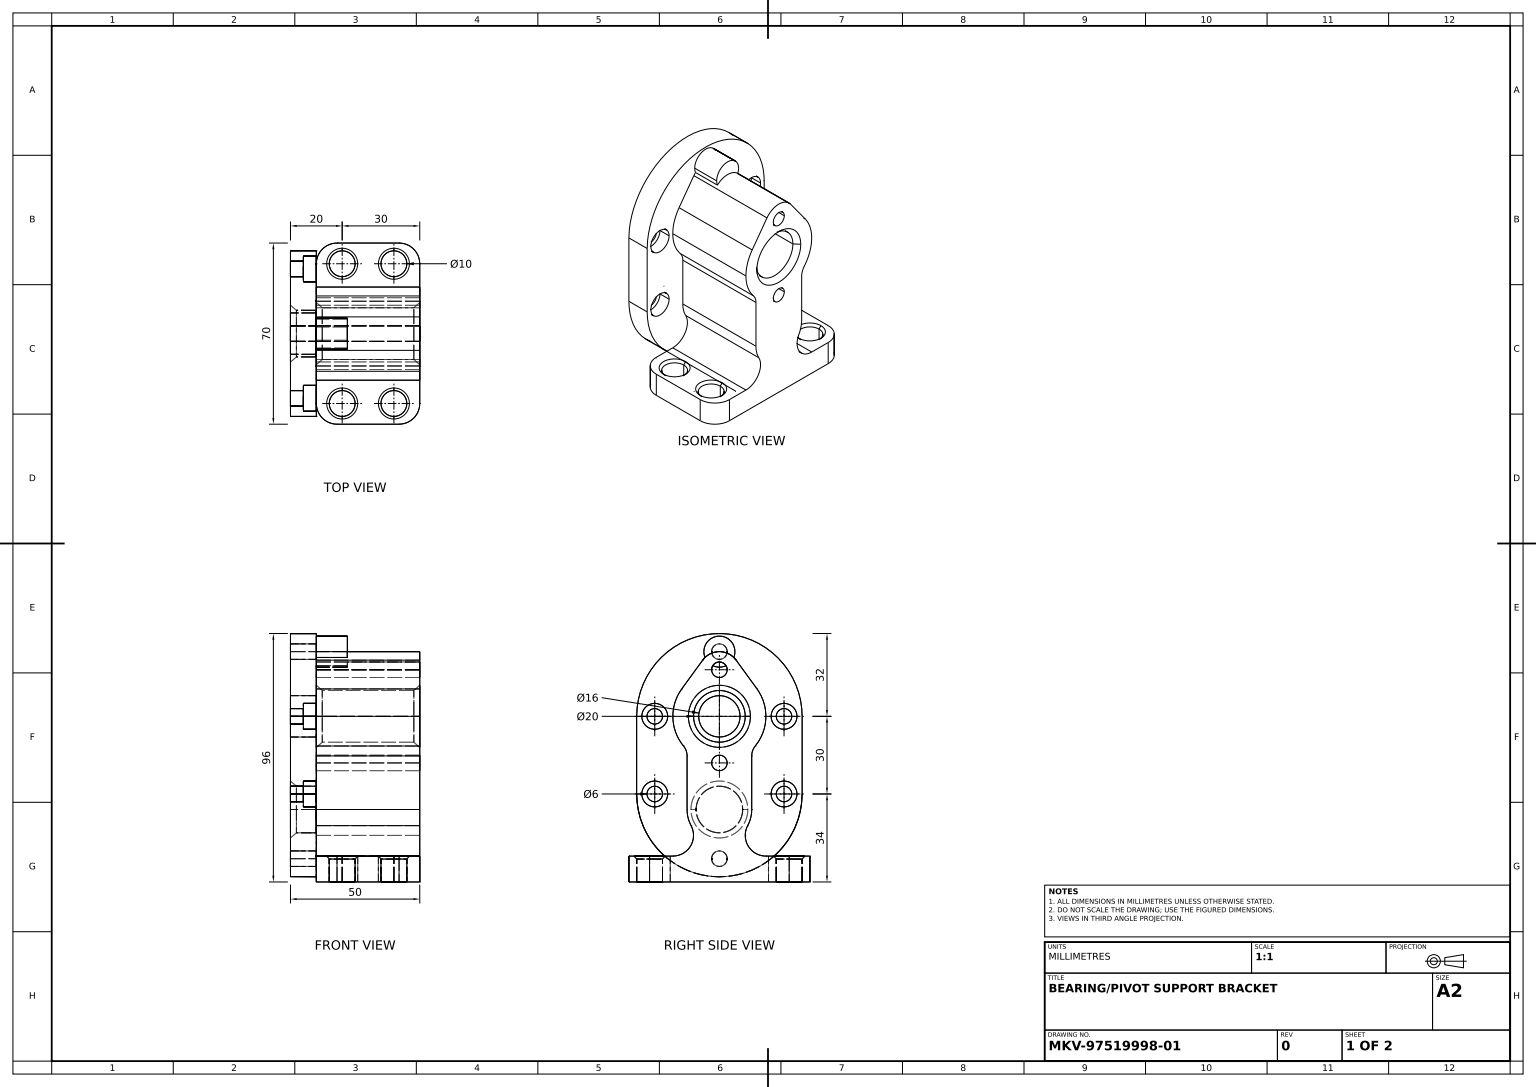
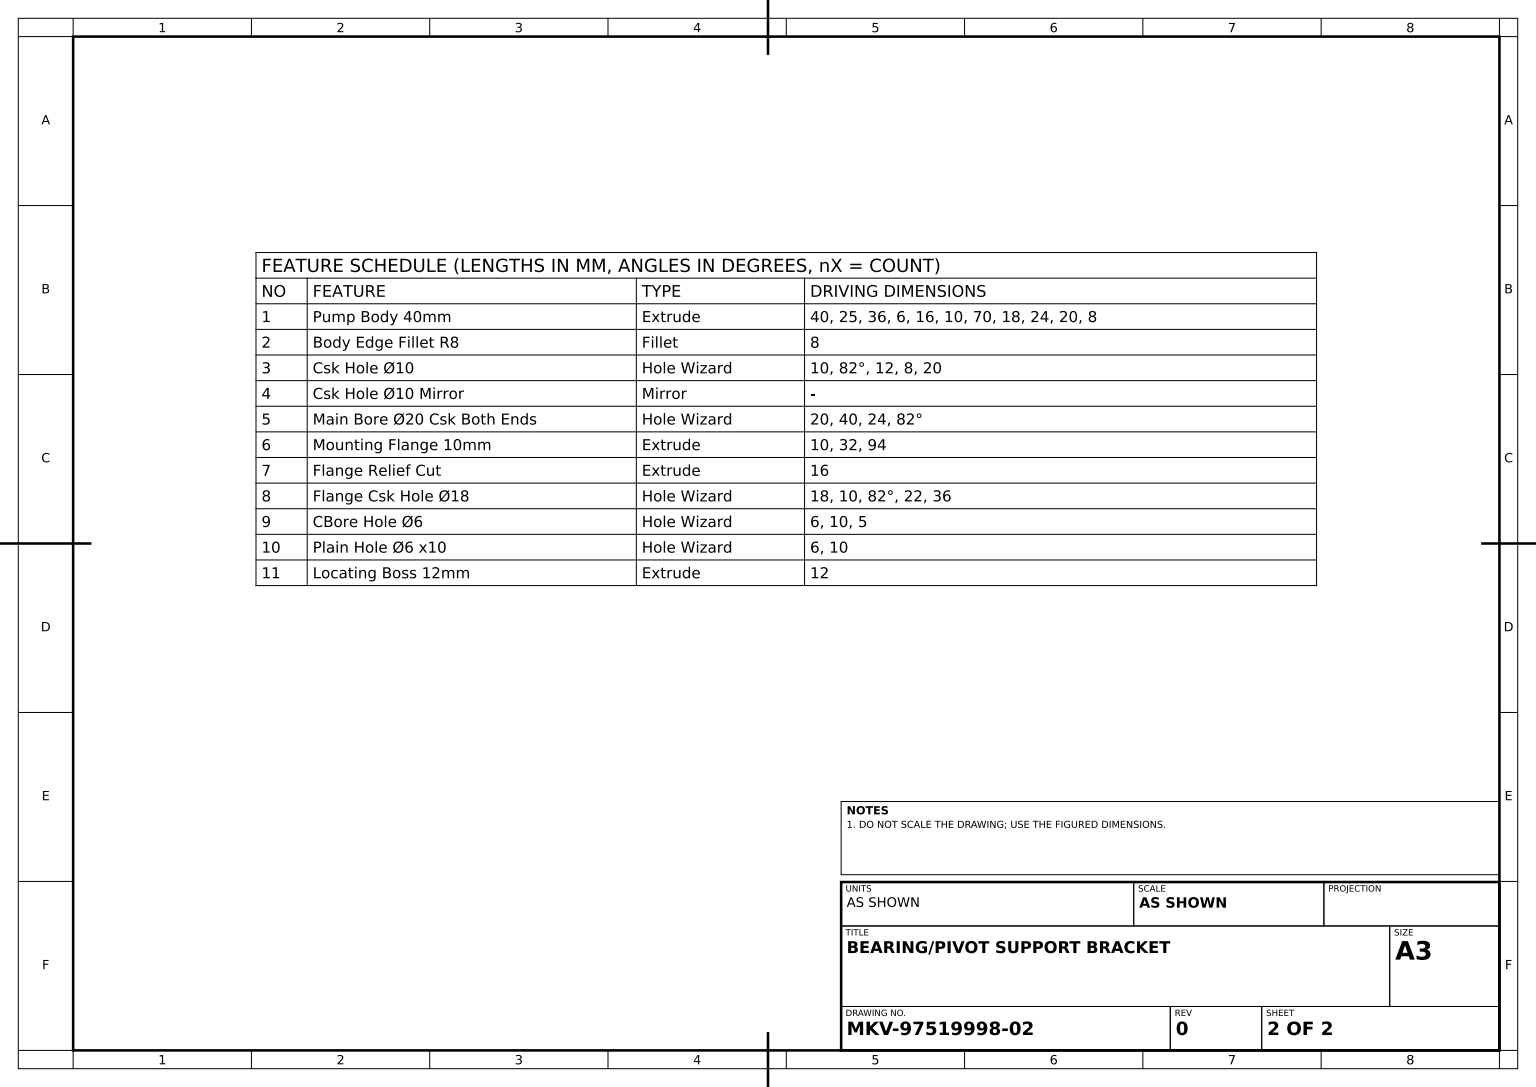
solid
v1 (8,-64,35)
v2 (0,-64,27)
e1 v1 v2 CIRCLE(AX(P(8,-64,27),D(0,-1,0),D(0,0,1)),8)
v3 (8,-54,35)
e2 v3 v1 LINE
v4 (0,-54,27)
e3 v4 v3 CIRCLE(AX(P(8,-54,27),D(0,1,0),D(0,0,-1)),8)
e4 v2 v4 LINE
face CYL(AX(P(8,-54,27),D(0,-1,0),D(0,0,-1)),8) [-e1 -e2 -e3 -e4]
v5 (-5,-30,30)
v6 (-5,-30,20)
e5 v5 v6 CIRCLE(AX(P(-5,-30,25),D(1,0,0),D(0,0,-1)),5)
e6 v6 v5 CIRCLE(AX(P(-5,-30,25),D(1,0,0),D(0,0,-1)),5)
v7 (-5,-30,28)
v8 (-5,-30,22)
e7 v7 v8 CIRCLE(AX(P(-5,-30,25),D(1,0,0),D(0,0,-1)),3)
e8 v8 v7 CIRCLE(AX(P(-5,-30,25),D(1,0,0),D(0,0,-1)),3)
face PLANE(AX(P(-5,-27,25),D(-1,0,0),D(0,0,1))) rev [e5 e6] [-e7 -e8]
v9 (0,25,6)
v10 (0,22.75,5.562149)
e9 v9 v10 CIRCLE(AX(P(0,25,0),D(1,0,0),D(0,0,-1)),6)
v11 (12,22.75,5.562149)
e10 v10 v11 LINE
v12 (12,25,6)
e11 v12 v11 CIRCLE(AX(P(12,25,0),D(1,0,0),D(0,0,-1)),6)
e12 v12 v9 LINE
face CYL(AX(P(12,25,0),D(-1,0,0),D(0,0,1)),6) [e9 e10 -e11 e12]
v13 (10,-54,-33)
v14 (10,-54,-21)
e13 v13 v14 CIRCLE(AX(P(10,-54,-27),D(0,1,0),D(0,0,1)),6)
e14 v14 v13 CIRCLE(AX(P(10,-54,-27),D(0,1,0),D(0,0,1)),6)
v15 (30,-54,-21)
v16 (30,-54,-33)
e15 v15 v16 CIRCLE(AX(P(30,-54,-27),D(0,1,0),D(0,0,1)),6)
e16 v16 v15 CIRCLE(AX(P(30,-54,-27),D(0,1,0),D(0,0,1)),6)
v17 (8,-54,-35)
v18 (0,-54,-27)
e17 v17 v18 CIRCLE(AX(P(8,-54,-27),D(0,1,0),D(0,0,-1)),8)
v19 (0,-54,-21.16601)
e18 v18 v19 LINE
v20 (0,-54,-18)
e19 v20 v19 LINE
v21 (40,-54,-18)
e20 v21 v20 LINE
v22 (40,-54,-27)
e21 v22 v21 LINE
v23 (32,-54,-35)
e22 v22 v23 CIRCLE(AX(P(32,-54,-27),D(0,1,0),D(0,0,-1)),8)
e23 v23 v17 LINE
face PLANE(AX(P(40,-54,-35),D(0,-1,0),D(0,0,-1))) rev [-e13 -e14] [-e15 -e16] [e17 e18 -e19 -e20 -e21 e22 e23]
v24 (-10,0,32)
v25 (0,0,32)
e24 v24 v25 LINE
v26 (0,0,-32)
e25 v25 v26 CIRCLE(AX(P(0,0,0),D(-1,0,0),D(0,0,1)),32)
v27 (-10,0,-32)
e26 v27 v26 LINE
e27 v24 v27 CIRCLE(AX(P(-10,0,0),D(-1,0,0),D(0,0,1)),32)
face CYL(AX(P(-10,0,0),D(1,0,0),D(0,0,-1)),32) [e24 e25 -e26 -e27]
v28 (-10,-55,-3)
v29 (-10,-55,3)
e28 v28 v29 CIRCLE(AX(P(-10,-55,0),D(-1,0,0),D(0,0,1)),3)
v30 (0,-55,3)
e29 v29 v30 LINE
v31 (0,-55,-3)
e30 v30 v31 CIRCLE(AX(P(0,-55,0),D(1,0,0),D(0,0,-1)),3)
e31 v28 v31 LINE
face CYL(AX(P(0,-55,0),D(1,0,0),D(0,0,-1)),3) rev [e28 e29 e30 -e31]
v32 (10,-55.150368,22)
v33 (10,-55.150368,32)
e32 v32 v33 CIRCLE(AX(P(10,-55.150368,27),D(0,1,0),D(0,0,1)),5)
v34 (10,-54,21)
e33 v32 v34 LINE
v35 (10,-54,33)
e34 v34 v35 CIRCLE(AX(P(10,-54,27),D(0,1,0),D(0,0,1)),6)
e35 v33 v35 LINE
face CONE(AX(P(10,-54,27),D(0,1,0),D(0,0,1)),6,0.715584993) rev [-e32 e33 e34 -e35]
v36 (12,25,-6)
v37 (0,25,-6)
e36 v36 v37 LINE
e37 v37 v9 CIRCLE(AX(P(0,25,0),D(1,0,0),D(0,0,-1)),6)
e38 v36 v12 CIRCLE(AX(P(12,25,0),D(1,0,0),D(0,0,-1)),6)
face CYL(AX(P(12,25,0),D(-1,0,0),D(0,0,1)),6) [e36 e37 -e12 -e38]
v38 (-5,-30,-20)
v39 (-5,-30,-30)
e39 v38 v39 CIRCLE(AX(P(-5,-30,-25),D(1,0,0),D(0,0,-1)),5)
e40 v39 v38 CIRCLE(AX(P(-5,-30,-25),D(1,0,0),D(0,0,-1)),5)
v40 (-5,-30,-28)
v41 (-5,-30,-22)
e41 v40 v41 CIRCLE(AX(P(-5,-30,-25),D(1,0,0),D(0,0,-1)),3)
e42 v41 v40 CIRCLE(AX(P(-5,-30,-25),D(1,0,0),D(0,0,-1)),3)
face PLANE(AX(P(-5,-27,-25),D(-1,0,0),D(0,0,1))) rev [e39 e40] [-e41 -e42]
v42 (30,-55.150368,-22)
e43 v42 v15 LINE
v43 (30,-55.150368,-32)
e44 v43 v42 CIRCLE(AX(P(30,-55.150368,-27),D(0,1,0),D(0,0,1)),5)
e45 v43 v16 LINE
face CONE(AX(P(30,-54,-27),D(0,1,0),D(0,0,1)),6,0.715584993) rev [e16 -e43 -e44 e45]
v44 (40,0,12)
v45 (40,0,-12)
e46 v44 v45 CIRCLE(AX(P(40,0,0),D(1,0,0),D(0,0,-1)),12)
v46 (37.699263,0,-10)
e47 v46 v45 LINE
v47 (37.699263,0,10)
e48 v47 v46 CIRCLE(AX(P(37.699263,0,0),D(1,0,0),D(0,0,-1)),10)
e49 v47 v44 LINE
face CONE(AX(P(40,0,0),D(1,0,0),D(0,0,-1)),12,0.715584993) rev [e46 -e47 -e48 e49]
v48 (0,19.571429,2.555506)
v49 (0,19.571429,-2.555506)
e50 v48 v49 CIRCLE(AX(P(0,25,0),D(1,0,0),D(0,0,-1)),6)
v50 (12,19.571429,-2.555506)
e51 v50 v49 LINE
v51 (12,19.571429,2.555506)
e52 v51 v50 CIRCLE(AX(P(12,25,0),D(1,0,0),D(0,0,-1)),6)
e53 v48 v51 LINE
face CYL(AX(P(12,25,0),D(-1,0,0),D(0,0,1)),6) [e50 -e51 -e52 -e53]
v52 (40,-42.235294,-10.941176)
v53 (40,-36,-12.5)
e54 v52 v53 CIRCLE(AX(P(40,-36,0.75),D(1,0,0),D(0,0,1)),13.25)
v54 (0,-42.235294,-10.941176)
e55 v52 v54 LINE
v55 (0,-36,-12.5)
e56 v54 v55 CIRCLE(AX(P(0,-36,0.75),D(1,0,0),D(0,0,1)),13.25)
e57 v53 v55 LINE
face CYL(AX(P(40,-36,0.75),D(-1,0,0),D(0,0,1)),13.25) [-e54 e55 e56 -e57]
v56 (-10,-30,-28)
e58 v56 v40 LINE
v57 (-10,-30,-22)
e59 v57 v56 CIRCLE(AX(P(-10,-30,-25),D(1,0,0),D(0,0,-1)),3)
e60 v57 v41 LINE
face CYL(AX(P(0,-30,-25),D(1,0,0),D(0,0,-1)),3) rev [-e58 -e59 e60 e42]
v58 (40,-15.288885,12.5)
v59 (0,-15.288885,12.5)
e61 v58 v59 LINE
v60 (40,-11.466664,13.875)
e62 v60 v58 CIRCLE(AX(P(40,-15.288885,18.5),D(-1,0,0),D(0,0,-1)),6)
v61 (0,-11.466664,13.875)
e63 v60 v61 LINE
e64 v61 v59 CIRCLE(AX(P(0,-15.288885,18.5),D(-1,0,0),D(0,0,-1)),6)
face CYL(AX(P(40,-15.288885,18.5),D(-1,0,0),D(0,0,1)),6) rev [-e61 -e62 e63 e64]
v62 (0,0,-8)
v63 (-10,0,-8)
e65 v62 v63 LINE
v64 (-10,0,8)
e66 v63 v64 CIRCLE(AX(P(-10,0,0),D(-1,0,0),D(0,0,1)),8)
v65 (0,0,8)
e67 v65 v64 LINE
e68 v65 v62 CIRCLE(AX(P(0,0,0),D(1,0,0),D(0,0,1)),8)
face CYL(AX(P(40.001,0,0),D(-1,0,0),D(0,0,1)),8) rev [e65 e66 -e67 e68]
v66 (0,-30,-20)
e69 v38 v66 LINE
v67 (0,-30,-30)
e70 v39 v67 LINE
e71 v67 v66 CIRCLE(AX(P(0,-30,-25),D(1,0,0),D(0,0,-1)),5)
face CYL(AX(P(0,-30,-25),D(1,0,0),D(0,0,-1)),5) rev [-e69 -e40 e70 e71]
v68 (-5,0,28)
v69 (-5,0,22)
e72 v68 v69 CIRCLE(AX(P(-5,0,25),D(1,0,0),D(0,0,-1)),3)
e73 v69 v68 CIRCLE(AX(P(-5,0,25),D(1,0,0),D(0,0,-1)),3)
v70 (-5,0,30)
v71 (-5,0,20)
e74 v70 v71 CIRCLE(AX(P(-5,0,25),D(1,0,0),D(0,0,-1)),5)
e75 v71 v70 CIRCLE(AX(P(-5,0,25),D(1,0,0),D(0,0,-1)),5)
face PLANE(AX(P(-5,3,25),D(-1,0,0),D(0,0,1))) rev [-e72 -e73] [e74 e75]
v72 (40,-64,27)
v73 (32,-64,35)
e76 v72 v73 CIRCLE(AX(P(32,-64,27),D(0,-1,0),D(0,0,1)),8)
v74 (40,-54,27)
e77 v74 v72 LINE
v75 (32,-54,35)
e78 v75 v74 CIRCLE(AX(P(32,-54,27),D(0,1,0),D(0,0,-1)),8)
e79 v73 v75 LINE
face CYL(AX(P(32,-15.288885,27),D(0,1,0),D(0,0,1)),8) [-e76 -e77 -e78 -e79]
v76 (-10,-30,28)
e80 v76 v7 LINE
v77 (-10,-30,22)
e81 v77 v76 CIRCLE(AX(P(-10,-30,25),D(1,0,0),D(0,0,-1)),3)
e82 v77 v8 LINE
face CYL(AX(P(0,-30,25),D(1,0,0),D(0,0,-1)),3) rev [-e80 -e81 e82 e8]
v78 (0,0,20)
e83 v71 v78 LINE
v79 (0,0,30)
e84 v70 v79 LINE
e85 v79 v78 CIRCLE(AX(P(0,0,25),D(1,0,0),D(0,0,-1)),5)
face CYL(AX(P(0,0,25),D(1,0,0),D(0,0,-1)),5) rev [-e83 -e74 e84 e85]
v80 (40,21.705882,-6.469519)
v81 (0,21.705882,-6.469519)
e86 v80 v81 LINE
v82 (40,10.588235,-14.556417)
e87 v82 v80 LINE
v83 (0,10.588235,-14.556417)
e88 v82 v83 LINE
e89 v83 v81 LINE
face PLANE(AX(P(40,10.588235,-14.556417),D(0,-0.588235294,0.808689829),D(0,-0.808689829,-0.588235294))) rev [-e86 -e87 e88 e89]
v84 (0,0,-20)
v85 (0,0,-30)
e90 v84 v85 CIRCLE(AX(P(0,0,-25),D(1,0,0),D(0,0,-1)),5)
e91 v85 v84 CIRCLE(AX(P(0,0,-25),D(1,0,0),D(0,0,-1)),5)
e92 v78 v79 CIRCLE(AX(P(0,0,25),D(1,0,0),D(0,0,-1)),5)
e93 v66 v67 CIRCLE(AX(P(0,-30,-25),D(1,0,0),D(0,0,-1)),5)
v86 (0,10.588235,14.556417)
v87 (0,0,18)
e94 v86 v87 CIRCLE(AX(P(0,0,0),D(1,0,0),D(0,0,-1)),18)
v88 (0,21.705882,6.469519)
e95 v88 v86 LINE
e96 v10 v88 CIRCLE(AX(P(0,17,0),D(1,0,0),D(0,0,-1)),8)
v89 (0,22.75,-5.562149)
e97 v89 v37 CIRCLE(AX(P(0,25,0),D(1,0,0),D(0,0,-1)),6)
e98 v81 v89 CIRCLE(AX(P(0,17,0),D(1,0,0),D(0,0,-1)),8)
v90 (0,-11.466664,-13.875)
e99 v90 v83 CIRCLE(AX(P(0,0,0),D(1,0,0),D(0,0,-1)),18)
v91 (0,-15.288885,-12.5)
e100 v91 v90 CIRCLE(AX(P(0,-15.288885,-18.5),D(-1,0,0),D(0,0,1)),6)
e101 v55 v91 LINE
v92 (0,-46,-10)
e102 v92 v54 CIRCLE(AX(P(0,-46,-18),D(-1,0,0),D(0,0,1)),8)
e103 v20 v92 CIRCLE(AX(P(0,-46,-18),D(-1,0,0),D(0,0,1)),8)
v93 (0,-30,-32)
e104 v93 v19 CIRCLE(AX(P(0,-30,0),D(-1,0,0),D(0,0,1)),32)
e105 v26 v93 LINE
v94 (0,-30,32)
e106 v94 v25 LINE
v95 (0,-54,21.16601)
e107 v95 v94 CIRCLE(AX(P(0,-30,0),D(-1,0,0),D(0,0,1)),32)
v96 (0,-54,18)
e108 v96 v95 LINE
v97 (0,-42.235294,10.941176)
e109 v97 v96 CIRCLE(AX(P(0,-46,18),D(-1,0,0),D(0,0,-1)),8)
v98 (0,-36,12.5)
e110 v98 v97 CIRCLE(AX(P(0,-36,-0.75),D(1,0,0),D(0,0,-1)),13.25)
e111 v59 v98 LINE
e112 v87 v61 CIRCLE(AX(P(0,0,0),D(1,0,0),D(0,0,-1)),18)
v99 (0,-30,20)
v100 (0,-30,30)
e113 v99 v100 CIRCLE(AX(P(0,-30,25),D(1,0,0),D(0,0,-1)),5)
e114 v100 v99 CIRCLE(AX(P(0,-30,25),D(1,0,0),D(0,0,-1)),5)
face PLANE(AX(P(0,0,0),D(-1,0,0),D(0,0,1))) rev [-e90 -e91] [-e85 -e92] [-e93 -e71] [-e94 -e95 -e96 -e9 -e37 -e97 -e98 -e89 -e99 -e100 -e101 -e56 -e102 -e103 e19 -e104 -e105 -e25 -e106 -e107 -e108 -e109 -e110 -e111 -e64 -e112] [-e113 -e114]
v101 (-10,-30,-32)
e115 v101 v93 LINE
e116 v27 v101 LINE
face PLANE(AX(P(-10,0,-32),D(0,0,1),D(0,-1,0))) rev [e105 -e115 -e116 e26]
v102 (-5,0,-28)
v103 (-5,0,-22)
e117 v102 v103 CIRCLE(AX(P(-5,0,-25),D(1,0,0),D(0,0,-1)),3)
e118 v103 v102 CIRCLE(AX(P(-5,0,-25),D(1,0,0),D(0,0,-1)),3)
v104 (-5,0,-20)
v105 (-5,0,-30)
e119 v104 v105 CIRCLE(AX(P(-5,0,-25),D(1,0,0),D(0,0,-1)),5)
e120 v105 v104 CIRCLE(AX(P(-5,0,-25),D(1,0,0),D(0,0,-1)),5)
face PLANE(AX(P(-5,3,-25),D(-1,0,0),D(0,0,1))) rev [-e117 -e118] [e119 e120]
v106 (40,-15.288885,-12.5)
e121 v106 v91 LINE
e122 v53 v106 LINE
face PLANE(AX(P(40,-15.288885,-12.5),D(0,0,1),D(0,-1,0))) rev [e57 e101 -e121 -e122]
v107 (10,-55.150368,-32)
v108 (10,-55.150368,-22)
e123 v107 v108 CIRCLE(AX(P(10,-55.150368,-27),D(0,1,0),D(0,0,1)),5)
v109 (10,-64,-22)
e124 v109 v108 LINE
v110 (10,-64,-32)
e125 v110 v109 CIRCLE(AX(P(10,-64,-27),D(0,1,0),D(0,0,1)),5)
e126 v110 v107 LINE
face CYL(AX(P(10,-54,-27),D(0,1,0),D(0,0,1)),5) rev [e123 -e124 -e125 e126]
v111 (2.300737,0,10)
e127 v111 v47 LINE
v112 (2.300737,0,-10)
e128 v112 v46 LINE
e129 v111 v112 CIRCLE(AX(P(2.300737,0,0),D(1,0,0),D(0,0,-1)),10)
face CYL(AX(P(40,0,0),D(1,0,0),D(0,0,-1)),10) rev [e127 e48 -e128 -e129]
v113 (30,-54,33)
v114 (30,-54,21)
e130 v113 v114 CIRCLE(AX(P(30,-54,27),D(0,1,0),D(0,0,1)),6)
v115 (30,-55.150368,22)
e131 v115 v114 LINE
v116 (30,-55.150368,32)
e132 v116 v115 CIRCLE(AX(P(30,-55.150368,27),D(0,1,0),D(0,0,1)),5)
e133 v116 v113 LINE
face CONE(AX(P(30,-54,27),D(0,1,0),D(0,0,1)),6,0.715584993) rev [e130 -e131 -e132 e133]
v117 (40,-18,3)
v118 (0,-18,3)
e134 v117 v118 LINE
v119 (0,-18,-3)
e135 v119 v118 CIRCLE(AX(P(0,-18,0),D(1,0,0),D(0,0,-1)),3)
v120 (40,-18,-3)
e136 v120 v119 LINE
e137 v120 v117 CIRCLE(AX(P(40,-18,0),D(1,0,0),D(0,0,-1)),3)
face CYL(AX(P(40,-18,0),D(-1,0,0),D(0,0,1)),3) rev [e134 -e135 -e136 e137]
face CYL(AX(P(0,-30,-25),D(1,0,0),D(0,0,-1)),5) rev [e69 e93 -e70 -e39]
v121 (-10,-30,32)
e138 v121 v24 LINE
e139 v121 v94 LINE
face PLANE(AX(P(-10,0,32),D(0,0,-1),D(0,1,0))) rev [-e24 -e138 e139 e106]
e140 v101 v121 CIRCLE(AX(P(-10,-30,0),D(-1,0,0),D(0,0,1)),32)
e141 v19 v95 CIRCLE(AX(P(0,-30,0),D(-1,0,0),D(0,0,1)),32)
face CYL(AX(P(-10,-30,0),D(1,0,0),D(0,0,-1)),32) [-e139 -e140 e115 e104 e141 e107]
e142 v105 v85 LINE
e143 v104 v84 LINE
face CYL(AX(P(0,0,-25),D(1,0,0),D(0,0,-1)),5) rev [e90 -e142 -e119 e143]
v122 (40,-11.466664,-13.875)
e144 v122 v90 LINE
e145 v106 v122 CIRCLE(AX(P(40,-15.288885,-18.5),D(-1,0,0),D(0,0,1)),6)
face CYL(AX(P(40,-15.288885,-18.5),D(-1,0,0),D(0,0,1)),6) rev [e100 -e144 -e145 e121]
e146 v5 v100 LINE
e147 v6 v99 LINE
face CYL(AX(P(0,-30,25),D(1,0,0),D(0,0,-1)),5) rev [-e146 -e6 e147 e113]
e148 v50 v51 CIRCLE(AX(P(12,18,0),D(1,0,0),D(0,0,-1)),3)
face PLANE(AX(P(12,25,0),D(1,0,0),D(0,0,-1))) [e148 e52]
e149 v108 v107 CIRCLE(AX(P(10,-55.150368,-27),D(0,1,0),D(0,0,1)),5)
e150 v108 v14 LINE
e151 v107 v13 LINE
face CONE(AX(P(10,-54,-27),D(0,1,0),D(0,0,1)),6,0.715584993) rev [-e149 e150 e14 -e151]
v123 (0,0,-12)
e152 v112 v123 LINE
v124 (0,0,12)
e153 v124 v123 CIRCLE(AX(P(0,0,0),D(1,0,0),D(0,0,-1)),12)
e154 v111 v124 LINE
face CONE(AX(P(2.300737,0,0),D(-1,0,0),D(0,0,1)),10,0.715584993) rev [e129 e152 -e153 -e154]
e155 v112 v111 CIRCLE(AX(P(2.300737,0,0),D(1,0,0),D(0,0,-1)),10)
e156 v46 v47 CIRCLE(AX(P(37.699263,0,0),D(1,0,0),D(0,0,-1)),10)
face CYL(AX(P(40,0,0),D(1,0,0),D(0,0,-1)),10) rev [-e155 e128 e156 -e127]
v125 (40,18,-3)
v126 (0,18,-3)
e157 v125 v126 LINE
v127 (0,18,3)
e158 v127 v126 CIRCLE(AX(P(0,18,0),D(1,0,0),D(0,0,-1)),3)
v128 (40,18,3)
e159 v128 v127 LINE
e160 v128 v125 CIRCLE(AX(P(40,18,0),D(1,0,0),D(0,0,-1)),3)
face CYL(AX(P(40,18,0),D(-1,0,0),D(0,0,1)),3) rev [e157 -e158 -e159 e160]
v129 (40,-46,-10)
e161 v129 v92 LINE
e162 v129 v52 CIRCLE(AX(P(40,-46,-18),D(-1,0,0),D(0,0,1)),8)
face CYL(AX(P(40,-46,-18),D(-1,0,0),D(0,0,1)),8) rev [e161 e102 -e55 -e162]
v130 (-10,0,-22)
e163 v130 v103 LINE
v131 (-10,0,-28)
e164 v131 v130 CIRCLE(AX(P(-10,0,-25),D(1,0,0),D(0,0,-1)),3)
e165 v131 v102 LINE
face CYL(AX(P(0,0,-25),D(1,0,0),D(0,0,-1)),3) rev [e117 -e163 -e164 e165]
v132 (40,10.588235,14.556417)
e166 v132 v86 LINE
v133 (40,21.705882,6.469519)
e167 v133 v132 LINE
e168 v133 v88 LINE
face PLANE(AX(P(40,10.588235,14.556417),D(0,-0.588235294,-0.808689829),D(0,0.808689829,-0.588235294))) rev [e95 -e166 -e167 e168]
v134 (40,-64,-27)
e169 v134 v22 LINE
v135 (32,-64,-35)
e170 v135 v134 CIRCLE(AX(P(32,-64,-27),D(0,-1,0),D(0,0,1)),8)
e171 v23 v135 LINE
face CYL(AX(P(32,-15.288885,-27),D(0,-1,0),D(0,0,-1)),8) [-e169 -e170 -e171 -e22]
v136 (30,-64,22)
v137 (30,-64,32)
e172 v136 v137 CIRCLE(AX(P(30,-64,27),D(0,1,0),D(0,0,1)),5)
e173 v136 v115 LINE
e174 v115 v116 CIRCLE(AX(P(30,-55.150368,27),D(0,1,0),D(0,0,1)),5)
e175 v137 v116 LINE
face CYL(AX(P(30,-54,27),D(0,1,0),D(0,0,1)),5) rev [-e172 e173 e174 -e175]
e176 v76 v77 CIRCLE(AX(P(-10,-30,25),D(1,0,0),D(0,0,-1)),3)
face CYL(AX(P(0,-30,25),D(1,0,0),D(0,0,-1)),3) rev [-e82 -e176 e80 e7]
e177 v29 v28 CIRCLE(AX(P(-10,-55,0),D(-1,0,0),D(0,0,1)),3)
e178 v31 v30 CIRCLE(AX(P(0,-55,0),D(1,0,0),D(0,0,-1)),3)
face CYL(AX(P(0,-55,0),D(1,0,0),D(0,0,-1)),3) rev [e177 e31 e178 -e29]
face PLANE(AX(P(0,-52,0),D(1,0,0),D(0,0,-1))) rev [-e30 -e178]
v138 (12,22.75,-5.562149)
e179 v138 v36 CIRCLE(AX(P(12,25,0),D(1,0,0),D(0,0,-1)),6)
e180 v138 v89 LINE
face CYL(AX(P(12,25,0),D(-1,0,0),D(0,0,1)),6) [-e36 -e179 e180 e97]
e181 v80 v133 CIRCLE(AX(P(40,17,0),D(1,0,0),D(0,0,-1)),8)
e182 v138 v11 CIRCLE(AX(P(12,17,0),D(1,0,0),D(0,0,-1)),8)
face CYL(AX(P(40,17,0),D(-1,0,0),D(0,0,1)),8) [e96 -e168 -e181 e86 e98 -e180 e182 -e10]
v139 (0,25,3)
v140 (0,25,-3)
e183 v139 v140 CIRCLE(AX(P(0,25,0),D(1,0,0),D(0,0,-1)),3)
e184 v140 v139 CIRCLE(AX(P(0,25,0),D(1,0,0),D(0,0,-1)),3)
face PLANE(AX(P(0,28,0),D(1,0,0),D(0,0,-1))) rev [-e183 -e184]
v141 (40,0,18)
e185 v141 v60 CIRCLE(AX(P(40,0,0),D(1,0,0),D(0,0,-1)),18)
e186 v141 v87 LINE
face CYL(AX(P(40,0,0),D(-1,0,0),D(0,0,1)),18) [-e63 -e185 e186 e112]
e187 v132 v141 CIRCLE(AX(P(40,0,0),D(1,0,0),D(0,0,-1)),18)
face CYL(AX(P(40,0,0),D(-1,0,0),D(0,0,1)),18) [-e186 -e187 e166 e94]
v142 (-10,25,-3)
e188 v142 v140 LINE
v143 (-10,25,3)
e189 v143 v139 LINE
e190 v143 v142 CIRCLE(AX(P(-10,25,0),D(-1,0,0),D(0,0,1)),3)
face CYL(AX(P(0,25,0),D(1,0,0),D(0,0,-1)),3) rev [e188 e184 -e189 e190]
e191 v114 v113 CIRCLE(AX(P(30,-54,27),D(0,1,0),D(0,0,1)),6)
face CONE(AX(P(30,-54,27),D(0,1,0),D(0,0,1)),6,0.715584993) rev [e191 -e133 -e174 e131]
e192 v62 v65 CIRCLE(AX(P(0,0,0),D(1,0,0),D(0,0,1)),8)
e193 v123 v124 CIRCLE(AX(P(0,0,0),D(1,0,0),D(0,0,-1)),12)
face PLANE(AX(P(0,0,0),D(-1,0,0),D(0,0,1))) rev [-e68 -e192] [e153 e193]
e194 v126 v49 CIRCLE(AX(P(0,18,0),D(1,0,0),D(0,0,-1)),3)
e195 v48 v127 CIRCLE(AX(P(0,18,0),D(1,0,0),D(0,0,-1)),3)
face PLANE(AX(P(0,0,0),D(-1,0,0),D(0,0,1))) rev [e194 -e50 e195 e158]
v144 (-0.202041,-36,9)
v145 (-0.202041,-36,-9)
e196 v144 v145 CIRCLE(AX(P(-0.202041,-36,0),D(-1,0,0),D(0,0,1)),9)
e197 v145 v144 CIRCLE(AX(P(-0.202041,-36,0),D(-1,0,0),D(0,0,1)),9)
face PLANE(AX(P(-0.202041,-36,0),D(1,0,0),D(0,0,-1))) rev [e196 e197]
v146 (10,-64,32)
e198 v146 v33 LINE
e199 v33 v32 CIRCLE(AX(P(10,-55.150368,27),D(0,1,0),D(0,0,1)),5)
v147 (10,-64,22)
e200 v147 v32 LINE
e201 v146 v147 CIRCLE(AX(P(10,-64,27),D(0,1,0),D(0,0,1)),5)
face CYL(AX(P(10,-54,27),D(0,1,0),D(0,0,1)),5) rev [e198 e199 -e200 -e201]
e202 v35 v34 CIRCLE(AX(P(10,-54,27),D(0,1,0),D(0,0,1)),6)
e203 v95 v4 LINE
e204 v75 v3 LINE
v148 (40,-54,18)
e205 v148 v74 LINE
e206 v148 v96 LINE
face PLANE(AX(P(40,-54,18),D(0,-1,0),D(0,0,-1))) rev [-e34 -e202] [e203 e3 -e204 e78 -e205 e206 e108] [-e130 -e191]
face CYL(AX(P(0,0,-25),D(1,0,0),D(0,0,-1)),5) rev [e91 -e143 -e120 e142]
e207 v125 v128 CIRCLE(AX(P(40,18,0),D(1,0,0),D(0,0,-1)),3)
face CYL(AX(P(40,18,0),D(-1,0,0),D(0,0,1)),3) rev [e207 e159 -e195 e53 -e148 e51 -e194 -e157]
e208 v118 v119 CIRCLE(AX(P(0,-18,0),D(1,0,0),D(0,0,-1)),3)
face PLANE(AX(P(0,0,0),D(-1,0,0),D(0,0,1))) rev [e208 e135]
e209 v73 v1 LINE
face PLANE(AX(P(40,-54,35),D(0,0,-1),D(-1,0,0))) rev [e79 e204 e2 -e209]
v149 (-7.699263,-36,-9)
e210 v145 v149 LINE
v150 (-7.699263,-36,9)
e211 v144 v150 LINE
e212 v150 v149 CIRCLE(AX(P(-7.699263,-36,0),D(-1,0,0),D(0,0,1)),9)
face CYL(AX(P(-10,-36,0),D(-1,0,0),D(0,0,1)),9) rev [-e210 -e196 e211 e212]
e213 v56 v57 CIRCLE(AX(P(-10,-30,-25),D(1,0,0),D(0,0,-1)),3)
face CYL(AX(P(0,-30,-25),D(1,0,0),D(0,0,-1)),3) rev [-e60 -e213 e58 e41]
v151 (30,-64,-32)
e214 v151 v43 LINE
v152 (30,-64,-22)
e215 v152 v42 LINE
e216 v151 v152 CIRCLE(AX(P(30,-64,-27),D(0,1,0),D(0,0,1)),5)
face CYL(AX(P(30,-54,-27),D(0,1,0),D(0,0,1)),5) rev [e214 e44 -e215 -e216]
face CONE(AX(P(10,-54,-27),D(0,1,0),D(0,0,1)),6,0.715584993) rev [-e150 -e123 e151 e13]
e217 v130 v131 CIRCLE(AX(P(-10,0,-25),D(1,0,0),D(0,0,-1)),3)
face CYL(AX(P(0,0,-25),D(1,0,0),D(0,0,-1)),3) rev [e163 e118 -e165 -e217]
face CYL(AX(P(0,-30,25),D(1,0,0),D(0,0,-1)),5) rev [-e5 e146 e114 -e147]
v153 (40,-42.235294,10.941176)
e218 v153 v97 LINE
v154 (40,-36,12.5)
e219 v154 v153 CIRCLE(AX(P(40,-36,-0.75),D(1,0,0),D(0,0,-1)),13.25)
e220 v154 v98 LINE
face CYL(AX(P(40,-36,-0.75),D(-1,0,0),D(0,0,1)),13.25) [-e218 -e219 e220 e110]
e221 v58 v154 LINE
face PLANE(AX(P(40,-15.288885,12.5),D(0,0,-1),D(0,1,0))) rev [-e220 -e221 e61 e111]
v155 (-10,0,28)
e222 v155 v68 LINE
v156 (-10,0,22)
e223 v156 v155 CIRCLE(AX(P(-10,0,25),D(1,0,0),D(0,0,-1)),3)
e224 v156 v69 LINE
face CYL(AX(P(0,0,25),D(1,0,0),D(0,0,-1)),3) rev [e73 -e222 -e223 e224]
e225 v64 v63 CIRCLE(AX(P(-10,0,0),D(-1,0,0),D(0,0,1)),8)
face CYL(AX(P(40.001,0,0),D(-1,0,0),D(0,0,1)),8) rev [-e65 e192 e67 e225]
e226 v117 v120 CIRCLE(AX(P(40,-18,0),D(1,0,0),D(0,0,-1)),3)
e227 v122 v82 CIRCLE(AX(P(40,0,0),D(1,0,0),D(0,0,-1)),18)
e228 v153 v148 CIRCLE(AX(P(40,-46,18),D(-1,0,0),D(0,0,-1)),8)
e229 v72 v134 LINE
e230 v21 v129 CIRCLE(AX(P(40,-46,-18),D(-1,0,0),D(0,0,1)),8)
e231 v45 v44 CIRCLE(AX(P(40,0,0),D(1,0,0),D(0,0,-1)),12)
face PLANE(AX(P(40,-15.288885,18.5),D(1,0,0),D(0,0,-1))) [-e226 -e137] [e54 e122 e145 e227 e87 e181 e167 e187 e185 e62 e221 e219 e228 e205 e77 e229 e169 e21 e230 e162] [-e231 -e46] [-e160 -e207]
v157 (0,-64,-27)
e232 v18 v157 LINE
e233 v2 v157 LINE
face PLANE(AX(P(0,-15.288885,18.5),D(1,0,0),D(0,0,-1))) rev [-e141 -e18 e232 -e233 e4 -e203]
e234 v147 v146 CIRCLE(AX(P(10,-64,27),D(0,1,0),D(0,0,1)),5)
face CYL(AX(P(10,-54,27),D(0,1,0),D(0,0,1)),5) rev [-e198 -e234 e200 e32]
face CONE(AX(P(40,0,0),D(1,0,0),D(0,0,-1)),12,0.715584993) rev [-e49 -e156 e47 e231]
e235 v149 v150 CIRCLE(AX(P(-7.699263,-36,0),D(-1,0,0),D(0,0,1)),9)
v158 (-10,-36,-11)
e236 v149 v158 LINE
v159 (-10,-36,11)
e237 v158 v159 CIRCLE(AX(P(-10,-36,0),D(-1,0,0),D(0,0,1)),11)
e238 v150 v159 LINE
face CONE(AX(P(-10,-36,0),D(-1,0,0),D(0,0,1)),11,0.715584993) rev [-e235 e236 e237 -e238]
v160 (8,-64,-35)
e239 v160 v17 LINE
e240 v157 v160 CIRCLE(AX(P(8,-64,-27),D(0,-1,0),D(0,0,1)),8)
face CYL(AX(P(8,-64,-27),D(0,1,0),D(0,0,1)),8) [-e232 -e17 -e239 -e240]
e241 v109 v110 CIRCLE(AX(P(10,-64,-27),D(0,1,0),D(0,0,1)),5)
e242 v137 v136 CIRCLE(AX(P(30,-64,27),D(0,1,0),D(0,0,1)),5)
e243 v152 v151 CIRCLE(AX(P(30,-64,-27),D(0,1,0),D(0,0,1)),5)
e244 v135 v160 LINE
face PLANE(AX(P(40,-64,35),D(0,1,0),D(0,0,1))) rev [e125 e241] [e172 e242] [e216 e243] [e234 e201] [e240 -e244 e170 -e229 e76 e209 e1 e233]
face CYL(AX(P(-10,-36,0),D(-1,0,0),D(0,0,1)),9) rev [e235 -e211 -e197 e210]
e245 v42 v43 CIRCLE(AX(P(30,-55.150368,-27),D(0,1,0),D(0,0,1)),5)
face CONE(AX(P(30,-54,-27),D(0,1,0),D(0,0,1)),6,0.715584993) rev [-e245 e43 e15 -e45]
face CYL(AX(P(40,-18,0),D(-1,0,0),D(0,0,1)),3) rev [e226 e136 -e208 -e134]
face CONE(AX(P(2.300737,0,0),D(-1,0,0),D(0,0,1)),10,0.715584993) rev [e154 -e193 -e152 e155]
e246 v155 v156 CIRCLE(AX(P(-10,0,25),D(1,0,0),D(0,0,-1)),3)
face CYL(AX(P(0,0,25),D(1,0,0),D(0,0,-1)),3) rev [-e224 -e246 e222 e72]
e247 v142 v143 CIRCLE(AX(P(-10,25,0),D(-1,0,0),D(0,0,1)),3)
face CYL(AX(P(0,25,0),D(1,0,0),D(0,0,-1)),3) rev [e183 -e188 e247 e189]
face PLANE(AX(P(40,-64,-35),D(0,0,1),D(1,0,0))) rev [e244 e239 -e23 e171]
face CYL(AX(P(40,-46,18),D(-1,0,0),D(0,0,1)),8) rev [e109 -e206 -e228 e218]
face CYL(AX(P(0,0,25),D(1,0,0),D(0,0,-1)),5) rev [-e84 -e75 e83 e92]
face CYL(AX(P(30,-54,27),D(0,1,0),D(0,0,1)),5) rev [-e173 -e242 e175 e132]
e248 v159 v158 CIRCLE(AX(P(-10,-36,0),D(-1,0,0),D(0,0,1)),11)
face PLANE(AX(P(-10,0,0),D(-1,0,0),D(0,0,1))) [e164 e217] [e176 e81] [-e177 -e28] [e59 e213] [e27 e116 e140 e138] [-e237 -e248] [-e247 -e190] [e223 e246] [-e225 -e66]
face CYL(AX(P(30,-54,-27),D(0,1,0),D(0,0,1)),5) rev [e245 -e214 -e243 e215]
face CONE(AX(P(10,-54,27),D(0,1,0),D(0,0,1)),6,0.715584993) rev [e35 e202 -e33 -e199]
face CYL(AX(P(10,-54,-27),D(0,1,0),D(0,0,1)),5) rev [e149 -e126 -e241 e124]
face CYL(AX(P(40,0,0),D(-1,0,0),D(0,0,1)),18) [e99 -e88 -e227 e144]
face CONE(AX(P(-10,-36,0),D(-1,0,0),D(0,0,1)),11,0.715584993) rev [e238 e248 -e236 -e212]
face CYL(AX(P(40,-46,-18),D(-1,0,0),D(0,0,1)),8) rev [e103 -e161 -e230 e20]
face PLANE(AX(P(12,25,0),D(1,0,0),D(0,0,-1))) [e38 e11 -e182 e179]
